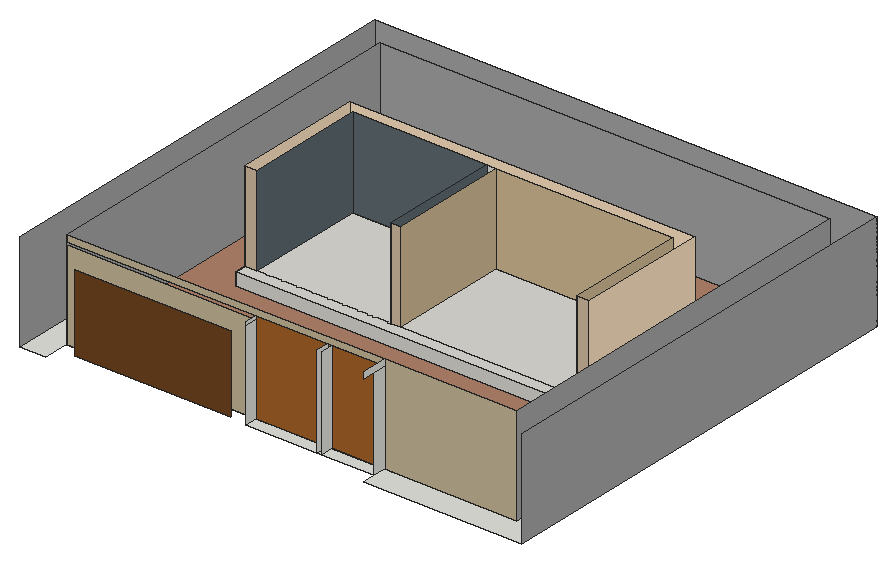
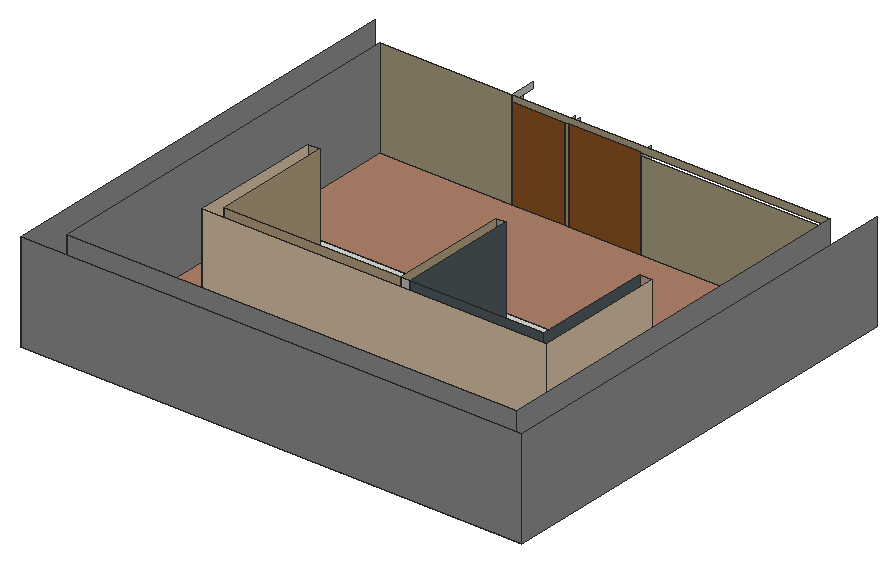
# SketchUp Ruby script. Lengths in inches.
U = 1.inch
M = Sketchup.active_model
def pt(a) = Geom::Point3d.new(a.map { |v| v * U })
def face(e, loops, mat)
  f = e.add_face(loops[0].map { |a| pt(a) })
  loops[1..].each { |l| e.add_face(l.map { |a| pt(a) }).erase! }
  f.material = f.back_material = mat if mat
  f
end
# faces: each face lists its corners as indices into pts; further lists are holes
def faces(e, pts, list, mat = nil) = list.each { |f| face(e, (f[0].is_a?(Array) ? f : [f]).map { |l| l.map { |i| pts[i] } }, mat) }
# xy, xz, yz: faces in a plane at the given z, y or x. An outline is a flat list of corners, or four numbers for a rectangle; further outlines are holes
def ring(l) = l.size == 4 ? [[l[0], l[1]], [l[2], l[1]], [l[2], l[3]], [l[0], l[3]]] : l.each_slice(2).to_a
def flat(e, list, mat, &to3) = list.each { |f| face(e, (f[0].is_a?(Array) ? f : [f]).map { |l| ring(l).map { |u, v| to3.(u, v) } }, mat) }
def xy(e, z, list, mat = nil) = flat(e, list, mat) { |x, y| [x, y, z] }
def xz(e, y, list, mat = nil) = flat(e, list, mat) { |x, z| [x, y, z] }
def yz(e, x, list, mat = nil) = flat(e, list, mat) { |y, z| [x, y, z] }
def lines(e, pts, list) = list.each { |a, b| e.add_line(pt(pts[a]), pt(pts[b])) }
# prism: a flat outline (further loops are holes) pulled along v
def prism(e, loops, v, mat = nil)
  f = face(e, loops, mat); d = Geom::Vector3d.new(v.map { |x| x * U })
  f.pushpull(f.normal.samedirection?(d) ? d.length : -d.length)
end
def box(e, o, s, mat = nil) = prism(e, [[o, [o[0] + s[0], o[1], o[2]], [o[0] + s[0], o[1] + s[1], o[2]], [o[0], o[1] + s[1], o[2]]]], [0, 0, s[2]], mat)
def at(x, y, z, deg = 0) = Geom::Transformation.translation(pt([x, y, z])) * Geom::Transformation.rotation(ORIGIN, Z_AXIS, deg.degrees)
def axes(o, x, y, z) = Geom::Transformation.new([*x, 0, *y, 0, *z, 0, *pt(o).to_a, 1])
def part(name) = M.definitions.add(name)
# library, detail: a bought-in or finely detailed component or shape, given as its bounding box
def library(name, o, s) = part(name).tap { |d| box(d.entities, o, s) }
def detail(e, o, s) = box(e.add_group.entities, o, s)
def put(e, d, t, mat = nil) = e.add_instance(d, t).tap { |i| i.material = mat if mat }
def group(e, t, mat = nil) = e.add_group.tap { |g| g.transformation = t; g.material = mat if mat }.entities
root = M.entities
M.materials.add("[0012_Bisque]3").color = [255, 228, 196]
M.materials.add("[Formica Beige]").color = [211, 187, 149]
M.materials.add("[Formica Laminate Light]").color = [213, 189, 164]
M.materials.add("[Formica Speckled Grey]").color = [94, 105, 111]
M.materials.add("[Pavers Driveway Brick]1").color = [176, 130, 106]
M.materials.add("[Quartz Light Brown]").color = [199, 184, 152]
M.materials.add("[Stone Vein Gray]").color = [166, 165, 165]
M.materials.add("[Terrazzo Tile Light]").color = [219, 217, 210]
M.materials.add("[Wood Bamboo]").color = [165, 98, 40]
M.materials.add("[Wood Floor Light]").color = [204, 176, 127]
M.materials.add("[Wood Floor Parquet]").color = [112, 68, 30]
xy(root,0,[[0,184.11,0,598.41,469.67,598.41,469.67,184.11,321.5,184.11,321.5,208.28,445.5,208.28,445.5,574.25,24.17,574.25,24.17,184.11],[201.37,196.19,268.28,208.28],[268.28,196.19,272.19,208.28],[272.19,196.19,321.5,208.28],[65.97,353.23,388.14,487.49]])
xy(root,0,[[[24.17,208.28,445.5,574.25],[65.97,353.23,388.14,487.49]]],"[Pavers Driveway Brick]1")
xy(root,11.6875,[[65.97,364.57,65.97,487.49,388.14,487.49,388.14,364.57,376.86,364.57,376.86,476.15,77.31,476.15,77.31,364.57],[202.72,364.57,211.5,476.15]])
xy(root,11.6875,[[65.97,353.23,388.14,364.57],[77.31,364.57,202.72,476.15],[211.5,364.57,376.86,476.15]],"[Terrazzo Tile Light]")
xz(root,198.55,[[39.34,0,185.03,72.25]],"[Wood Floor Parquet]")
xz(root,208.28,[[24.17,0,201.37,83.1875],[321.5,0,445.5,92.125],[24.17,86.16,321.5,92.125]],"[Quartz Light Brown]")
xz(root,208.28,[[201.37,0,268.28,86.16],[272.19,0,321.5,86.16]],"[Wood Bamboo]")
xz(root,208.28,[[268.28,0,272.19,86.16]],"[Wood Floor Light]")
xz(root,353.23,[[65.97,0,388.14,11.6875]],"[Terrazzo Tile Light]")
xz(root,364.57,[[65.97,11.6875,77.31,95.625],[202.72,11.6875,211.5,95.625],[376.86,11.6875,388.14,95.625]],"[Formica Laminate Light]")
xz(root,476.15,[[202.72,11.6875,211.5,95.625]])
xz(root,476.15,[[211.5,11.6875,376.86,95.625]],"[Formica Beige]")
xz(root,476.15,[[77.31,11.6875,202.72,95.625]],"[Formica Speckled Grey]")
xz(root,487.49,[[65.97,11.6875,388.14,95.625]],"[0012_Bisque]3")
xz(root,487.49,[[65.97,0,388.14,11.6875]],"[Terrazzo Tile Light]")
xz(root,574.25,[[24.17,0,445.5,92.125]],"[Stone Vein Gray]")
xz(root,598.41,[[0,0,469.67,92.125]],"[Stone Vein Gray]")
yz(root,0,[[184.11,0,598.41,92.125]],"[Stone Vein Gray]")
yz(root,24.17,[[208.28,0,574.25,92.125]],"[Stone Vein Gray]")
yz(root,65.97,[[364.57,11.6875,487.49,95.625]],"[0012_Bisque]3")
yz(root,65.97,[[353.23,0,487.49,11.6875]],"[Terrazzo Tile Light]")
yz(root,77.31,[[364.57,11.6875,476.15,95.625]],"[Formica Speckled Grey]")
yz(root,201.37,[[196.19,0,208.28,83.1875],[196.19,83.1875,208.28,86.16]])
yz(root,202.72,[[364.57,11.6875,476.15,95.625]],"[Formica Speckled Grey]")
yz(root,211.5,[[364.57,11.6875,476.15,95.625]],"[Formica Beige]")
yz(root,268.28,[[196.19,0,208.28,86.16]])
yz(root,272.19,[[196.19,0,208.28,86.16]])
yz(root,321.5,[[196.19,0,208.28,86.16],[184.11,86.16,208.28,92.125]])
yz(root,376.86,[[364.57,11.6875,476.15,95.625]],"[Formica Beige]")
yz(root,388.14,[[364.57,11.6875,487.49,95.625]],"[0012_Bisque]3")
yz(root,388.14,[[353.23,0,487.49,11.6875]],"[Terrazzo Tile Light]")
yz(root,445.5,[[208.28,0,574.25,92.125]],"[Stone Vein Gray]")
yz(root,469.67,[[184.11,0,598.41,92.125]],"[Stone Vein Gray]")
